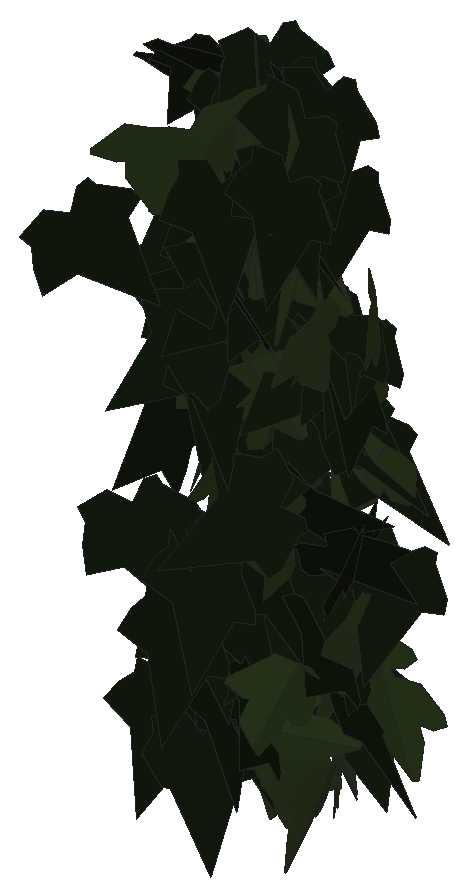
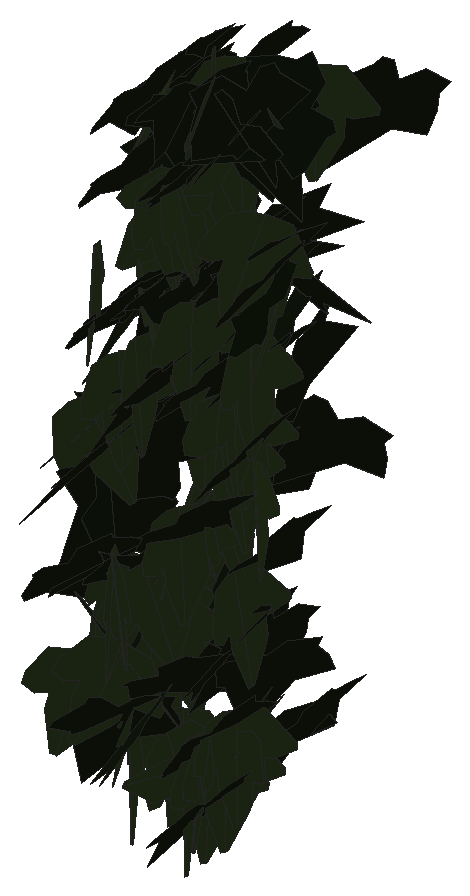
# SketchUp Ruby script. Lengths in inches.
U = 1.inch
M = Sketchup.active_model
def pt(a) = Geom::Point3d.new(a.map { |v| v * U })
def face(e, loops, mat)
  f = e.add_face(loops[0].map { |a| pt(a) })
  loops[1..].each { |l| e.add_face(l.map { |a| pt(a) }).erase! }
  f.material = f.back_material = mat if mat
  f
end
# faces: each face lists its corners as indices into pts; further lists are holes
def faces(e, pts, list, mat = nil) = list.each { |f| face(e, (f[0].is_a?(Array) ? f : [f]).map { |l| l.map { |i| pts[i] } }, mat) }
# xy, xz, yz: faces in a plane at the given z, y or x. An outline is a flat list of corners, or four numbers for a rectangle; further outlines are holes
def ring(l) = l.size == 4 ? [[l[0], l[1]], [l[2], l[1]], [l[2], l[3]], [l[0], l[3]]] : l.each_slice(2).to_a
def flat(e, list, mat, &to3) = list.each { |f| face(e, (f[0].is_a?(Array) ? f : [f]).map { |l| ring(l).map { |u, v| to3.(u, v) } }, mat) }
def xy(e, z, list, mat = nil) = flat(e, list, mat) { |x, y| [x, y, z] }
def xz(e, y, list, mat = nil) = flat(e, list, mat) { |x, z| [x, y, z] }
def yz(e, x, list, mat = nil) = flat(e, list, mat) { |y, z| [x, y, z] }
def lines(e, pts, list) = list.each { |a, b| e.add_line(pt(pts[a]), pt(pts[b])) }
# prism: a flat outline (further loops are holes) pulled along v
def prism(e, loops, v, mat = nil)
  f = face(e, loops, mat); d = Geom::Vector3d.new(v.map { |x| x * U })
  f.pushpull(f.normal.samedirection?(d) ? d.length : -d.length)
end
def box(e, o, s, mat = nil) = prism(e, [[o, [o[0] + s[0], o[1], o[2]], [o[0] + s[0], o[1] + s[1], o[2]], [o[0], o[1] + s[1], o[2]]]], [0, 0, s[2]], mat)
def at(x, y, z, deg = 0) = Geom::Transformation.translation(pt([x, y, z])) * Geom::Transformation.rotation(ORIGIN, Z_AXIS, deg.degrees)
def axes(o, x, y, z) = Geom::Transformation.new([*x, 0, *y, 0, *z, 0, *pt(o).to_a, 1])
def part(name) = M.definitions.add(name)
# library, detail: a bought-in or finely detailed component or shape, given as its bounding box
def library(name, o, s) = part(name).tap { |d| box(d.entities, o, s) }
def detail(e, o, s) = box(e.add_group.entities, o, s)
def put(e, d, t, mat = nil) = e.add_instance(d, t).tap { |i| i.material = mat if mat }
def group(e, t, mat = nil) = e.add_group.tap { |g| g.transformation = t; g.material = mat if mat }.entities
root = M.entities
M.materials.add("efeu1").color = [18, 25, 13]
M.materials.add("efeu2").color = [43, 57, 29]
c1 = part("ivyleaf_10")
p = [[0,0.5,-0.03],[-0.0625,2.02,-0.43],[-0.19,2.01,-0.46],[-0.54,1.05,-0.29],[-0.52,0.625,-0.18],[-0.83,0.76,-0.28],
  [-1.16,0.64,-0.33],[-1.15,0.33,-0.24],[-0.77,-0.39,0.02],[-0.3,-0.51,0.16],[0.04,-0.48,0.23],[-0.02,2.01,-0.4375],
  [-0.06,2.01,-0.43],[0.04,-0.49,0.23],[0.67,-0.49,0.14],[1.38,0.36,-0.2],[1.375,0.51,-0.24],[0.81,0.65,-0.19],
  [0.62,0.59,-0.15],[0.6,1.09,-0.28],[0.5,1.23,-0.31]]
faces(c1.entities,p,[[0,1,2,3,4,5,6,7,8,9,10],[11,12,0,13,14,15,16,17,18,19,20]],"efeu2")
c2 = part("ivyleaf_9")
p = [[1.54,2.16,1.25],[1.36,2.04,1.19],[-0.21,0.99,0.68],[-0.71,1.11,0.82],[-0.85,0.86,0.67],[-0.8,0.17,0.21],
  [-0.9,-0.01,0.1],[-0.67,-0.16,-0.02],[-0.08,-0.08,-0.05],[-0.03,-0.6,-0.4],[0.65,-0.88,-0.66],[0.83,-0.6,-0.49],
  [1.29,-0.42,-0.43],[1.8125,-0.07,-0.26],[1.21,0.44,0.15]]
faces(c2.entities,p,[[0,1,2,3,4,5,6,7,8,9,10,11,12,13,14]],"efeu1")
put(root,c1,axes([19.24,222.77,237.38],[0.17278,-0.38617,-0.2665],[-0.08276,0.25446,-0.42238],[0.46184,0.19007,0.02402]))
put(root,c2,axes([18.98,223.02,240.1],[0.03689,-0.49723,0.03738],[0.00276,-0.03728,-0.4986],[0.49863,0.03699,0]))
put(root,c1,axes([19.14,222.94,240.54],[-0.38375,-0.28732,-0.14208],[0.14647,0.03995,-0.47639],[0.28511,-0.40725,0.0535]))
put(root,c1,axes([19.23,223.1,236.16],[-0.02784,-0.49904,-0.01339],[0.00029,0.01339,-0.49982],[0.49922,-0.02784,-0.00046]))
put(root,c2,axes([18.89,222.41,241.98],[0.46915,0.04238,0.16764],[0.15648,0.10224,-0.46375],[-0.07359,0.4876,0.08267]))
put(root,c2,axes([19.27,222.8,240.12],[-0.27145,-0.32528,0.26553],[-0.08709,-0.2657,-0.41451],[0.41077,-0.27129,0.08759]))
put(root,c2,axes([19.43,222.72,242.08],[0.08196,0.35297,-0.34452],[-0.16723,-0.30867,-0.35603],[-0.46402,0.17359,0.06745]))
put(root,c1,axes([19.3,223.07,234.42],[-0.19485,-0.45862,-0.04129],[0.00891,0.04107,-0.49823],[0.46039,-0.1949,-0.00783]))
put(root,c2,axes([19.64,221.89,239.57],[-0.25149,0.23224,0.36444],[-0.31807,0.18598,-0.338],[-0.29255,-0.40184,0.05419]))
put(root,c2,axes([18.9,223.07,239.83],[0.23492,-0.30149,0.32236],[0.19362,-0.25778,-0.38218],[0.39664,0.30439,-0.00437]))
put(root,c1,axes([19.32,223.25,234.19],[-0.19054,-0.46002,-0.04561],[0.01084,0.04488,-0.49786],[0.46214,-0.19072,-0.00713]))
put(root,c2,axes([19.2,222.13,234.18],[-0.08276,-0.46166,0.17327],[-0.00631,-0.17469,-0.46845],[0.49306,-0.07972,0.02309]))
put(root,c1,axes([19.375,222.71,238.78],[-0.05874,-0.48909,-0.08565],[0.01706,0.0842,-0.49256],[0.49624,-0.06079,0.0068]))
put(root,c1,axes([19.51,222.18,239.29],[-0.08738,0.22127,0.43978],[-0.26336,0.35636,-0.23162],[-0.41594,-0.27212,0.05427]))
put(root,c2,axes([19.2,222.62,235.64],[0.14122,-0.29563,-0.37771],[-0.0462,0.38352,-0.31745],[0.47741,0.12456,0.081]))
put(root,c2,axes([19.24,222.63,235.18],[-0.0934,-0.44065,-0.21703],[0.05724,0.20965,-0.4503],[0.48785,-0.10896,0.01128]))
put(root,c1,axes([19.54,222.79,241.7],[-0.46424,-0.16739,0.08041],[-0.06712,-0.0506,-0.49288],[0.17314,-0.46842,0.02451]))
put(root,c2,axes([19.2,223.3125,235.59],[0.1715,-0.46778,-0.04208],[0.00756,0.04754,-0.49768],[0.46961,0.17007,0.02338]))
put(root,c2,axes([19.27,223.14,237.83],[-0.00405,-0.47425,0.15835],[0.02505,-0.15835,-0.4736],[0.49936,0.0041,0.02504]))
put(root,c2,axes([19.22,223.73,233.86],[0.16797,-0.44931,-0.1411],[0.02929,0.15948,-0.47298],[0.47003,0.15062,0.0799]))
put(root,c1,axes([19.54,221.43,241.57],[-0.40762,-0.28889,0.01977],[-0.01661,-0.01076,-0.49961],[0.28908,-0.40796,-0.00083]))
put(root,c1,axes([19.55,223.18,233.95],[-0.16684,-0.46113,-0.09759],[0.03236,0.09207,-0.49038],[0.47023,-0.16995,-0.00088]))
put(root,c1,axes([19.59,223.3,234.125],[0.28488,-0.29459,-0.28647],[-0.05686,0.31697,-0.38249],[0.40696,0.2505,0.1471]))
put(root,c2,axes([19.4,223.38,234.53],[-0.02239,-0.4995,0.00124],[-0.00344,-0.00109,-0.49999],[0.49949,-0.0224,-0.00339]))
put(root,c2,axes([19.41,220.2,241.14],[0.03149,-0.2267,-0.44454],[0.00486,0.44554,-0.22687],[0.49898,0.00997,0.03026]))
put(root,c1,axes([19.61,222.68,238.23],[0.06106,-0.48381,-0.11043],[0.01791,0.11334,-0.48666],[0.49593,0.05548,0.03117]))
put(root,c1,axes([19.55,222.72,241.24],[0.11348,0.48549,0.03771],[-0.04596,0.04922,-0.49544],[-0.48478,0.10898,0.0558]))
put(root,c2,axes([19.375,222.8125,234.2],[0.24582,-0.43247,-0.05045],[-0.00936,0.05267,-0.49713],[0.4353,0.24535,0.0178]))
put(root,c1,axes([19.77,222.54,237.92],[-0.43303,-0.23228,0.09238],[-0.07562,-0.0544,-0.49125],[0.23827,-0.43941,0.01198]))
put(root,c2,axes([19.41,222.92,241.8],[-0.18122,-0.09721,-0.45575],[0.39386,0.22941,-0.20554],[0.24907,-0.4335,-0.00657]))
put(root,c2,axes([19.47,222.6,235.58],[0.17757,-0.38809,-0.26049],[-0.05617,0.25891,-0.42404],[0.46402,0.17985,0.04835]))
put(root,c2,axes([19.58,222.3,236.23],[-0.10249,-0.4613,0.16341],[-0.02049,-0.16276,-0.47232],[0.48895,-0.10351,0.01446]))
put(root,c1,axes([19.72,223.4,233.85],[0.32472,-0.28577,-0.25078],[-0.07158,0.27795,-0.40941],[0.3734,0.3018,0.1396]))
put(root,c2,axes([19.52,222.65,239.96],[-0.01102,-0.49986,-0.00467],[0.00024,0.00466,-0.49998],[0.49988,-0.01102,0.00014]))
put(root,c2,axes([19.5625,222.9375,241.47],[0.02201,-0.47233,0.16255],[0.00914,-0.1623,-0.47284],[0.49943,0.02379,0.00149]))
put(root,c1,axes([19.82,222.4,237.33],[0.00796,-0.49503,-0.06988],[-0.01366,0.06965,-0.49494],[0.49975,0.00979,-0.01242]))
put(root,c2,axes([19.65,221.61,238.19],[0.0786,-0.17823,-0.46049],[0.3059,-0.34846,0.18709],[-0.38762,-0.31114,0.05426]))
put(root,c2,axes([19.51,221.875,238.9],[0.32,-0.38407,0.00967],[0.00641,-0.00725,-0.49991],[0.38414,0.32006,0.00028]))
put(root,c2,axes([19.63,222.4,238.52],[-0.03097,-0.48134,0.13171],[0.02916,-0.13348,-0.48097],[0.49819,-0.02211,0.03634]))
put(root,c2,axes([19.5625,222.56,234.29],[0.14424,-0.45462,0.15005],[0.02872,-0.14821,-0.47666],[0.47788,0.14613,-0.01664]))
put(root,c2,axes([19.67,222.09,233.92],[-0.07523,-0.47784,-0.12654],[0.0303,0.1233,-0.48361],[0.49338,-0.08043,0.01041]))
put(root,c2,axes([19.6,221,237.25],[-0.11147,-0.25925,-0.41275],[0.2764,0.31513,-0.27258],[0.40147,-0.28893,0.07305]))
put(root,c2,axes([19.83,223.42,236.98],[-0.22323,-0.42942,0.12557],[0.01525,-0.14755,-0.47749],[0.44714,-0.20935,0.07897]))
put(root,c1,axes([19.64,222.12,239.84],[-0.32479,0.06175,-0.3751],[0.34635,-0.15528,-0.32546],[-0.15669,-0.47125,0.0581]))
put(root,c2,axes([19.98,223.5,235.09],[-0.32862,-0.34969,0.14046],[-0.03433,-0.15781,-0.4732],[0.37528,-0.32064,0.07971]))
put(root,c1,axes([19.88,222.84,242.1],[-0.17244,0.40379,-0.23921],[0.07485,-0.22793,-0.43869],[-0.46332,-0.1871,0.01816]))
put(root,c1,axes([20.01,222.4,236.65],[0.0629,-0.48601,0.0992],[0.02876,-0.09625,-0.4898],[0.49519,0.06733,0.01584]))
put(root,c1,axes([19.88,223.01,233.77],[0.12226,0.01737,-0.48451],[0.21946,0.44357,0.07128],[0.43231,-0.23009,0.10084]))
put(root,c1,axes([20.03,222.17,241.58],[-0.04064,-0.42806,-0.25517],[0.0721,0.24827,-0.42798],[0.4931,-0.07158,0.04155]))
put(root,c1,axes([20.09,223.04,236.625],[-0.14708,-0.47659,-0.0351],[0.01122,0.03327,-0.49877],[0.47775,-0.1475,0.0009]))
put(root,c2,axes([19.94,222.94,238.45],[-0.10769,-0.46778,0.13995],[0.01987,-0.14739,-0.47737],[0.48786,-0.09725,0.05033]))
put(root,c2,axes([19.89,223,242.14],[0.04424,-0.45024,-0.21291],[0.02707,0.2156,-0.45031],[0.4973,0.02832,0.04346]))
put(root,c1,axes([20.05,222.08,240.57],[-0.42098,0.25796,-0.07898],[0.07309,-0.03184,-0.4936],[-0.25969,-0.42713,-0.0109]))
put(root,c1,axes([20.08,222.17,241.8],[-0.27717,-0.39435,-0.1329],[0.11239,0.08282,-0.48011],[0.40068,-0.29602,0.04273]))
put(root,c2,axes([20.12,222.04,239.7],[-0.21627,-0.32562,0.31177],[-0.02329,-0.33726,-0.36839],[0.45021,-0.17387,0.13071]))
put(root,c2,axes([20.05,222.95,241.85],[-0.19656,-0.40287,-0.22149],[0.11851,0.18834,-0.44775],[0.44421,-0.22852,0.02145]))
put(root,c1,axes([20.25,222.95,233.77],[-0.07528,-0.48543,0.09321],[-0.0002,-0.09426,-0.49103],[0.4943,-0.07396,0.014]))
put(root,c2,axes([20.3,221.33,239.46],[-0.22843,-0.319,0.30993],[-0.1806,-0.25188,-0.39235],[0.40645,-0.2912,-0.00015]))
put(root,c1,axes([20.31,222.57,238.875],[-0.16578,-0.46461,-0.08156],[0.01192,0.0823,-0.49304],[0.47157,-0.16541,-0.01621]))
put(root,c2,axes([20.01,222.85,241.08],[0.21018,-0.42419,-0.16091],[0.02326,0.18718,-0.46306],[0.45308,0.18716,0.09842]))
put(root,c2,axes([20.16,222.67,239.69],[-0.14333,-0.41614,0.23724],[0.036,-0.25629,-0.42781],[0.47766,-0.10556,0.10343]))
put(root,c1,axes([20.37,222.7,240.54],[0.05537,-0.49655,-0.01922],[-0.01086,0.01813,-0.49955],[0.49681,0.05574,-0.00878]))
put(root,c1,axes([20.43,223.17,235.89],[-0.22569,-0.42262,0.14302],[-0.02015,-0.15045,-0.4764],[0.44571,-0.2208,0.05088]))
put(root,c1,axes([20.49,222.5625,233.8],[-0.46566,-0.17103,0.06249],[-0.05953,-0.01918,-0.49607],[0.17208,-0.46945,-0.0025]))
put(root,c2,axes([20.15,223.65,234.47],[0.26996,-0.41961,-0.03238],[-0.01824,0.02676,-0.49895],[0.42046,0.27058,-0.00086]))
put(root,c2,axes([20.2,222.24,238.47],[0.08146,-0.49264,0.02591],[0.00732,-0.02505,-0.49932],[0.49327,0.08172,0.00313]))
put(root,c1,axes([20.45,222.89,240.53],[-0.08095,-0.49292,0.02187],[0.01292,-0.02427,-0.49924],[0.49324,-0.08026,0.01666]))
put(root,c2,axes([20.21,222.7,240.98],[0.08881,-0.47835,-0.11529],[0.01541,0.1198,-0.48519],[0.49181,0.08263,0.03602]))
put(root,c2,axes([20.28,221.53,239.11],[0.08663,-0.49143,0.03154],[0.00496,-0.03115,-0.499],[0.49241,0.08677,-0.00052]))
put(root,c1,axes([20.48,222.38,236.47],[0.14237,-0.36035,-0.31603],[0.04568,0.33838,-0.36526],[0.47712,0.07513,0.12927]))
put(root,c2,axes([20.31,222.67,239.52],[0.08382,-0.43797,-0.22617],[0.02808,0.23328,-0.44135],[0.49212,0.06129,0.06371]))
put(root,c2,axes([20.4,221.29,236.625],[-0.05643,-0.48836,0.09123],[0.02027,-0.09401,-0.49066],[0.49639,-0.05168,0.0304]))
put(root,c2,axes([20.4375,221.625,239.95],[0.44629,-0.0716,-0.21377],[-0.20932,0.04446,-0.45189],[0.08372,0.49285,0.00971]))
put(root,c1,axes([20.5625,221.86,237.63],[0.21074,-0.44521,0.08587],[0.02404,-0.08359,-0.49238],[0.45278,0.21166,-0.01383]))
put(root,c1,axes([20.57,223.52,236.12],[0.31223,-0.37642,-0.10404],[-0.00976,0.12563,-0.48386],[0.39041,0.30418,0.0711]))
put(root,c2,axes([20.36,222.34,236.25],[0.23697,-0.43101,-0.08987],[-0.02032,0.09124,-0.49118],[0.43981,0.23645,0.02573]))
put(root,c2,axes([20.39,223.03,238.43],[0.24888,-0.34968,-0.25648],[-0.06132,0.26436,-0.41994],[0.4293,0.24049,0.0887]))
put(root,c1,axes([20.64,223.48,235.95],[0.1365,-0.42725,-0.22097],[0.00098,0.22994,-0.44399],[0.48101,0.12077,0.06361]))
put(root,c2,axes([20.51,220.74,236.26],[-0.06199,-0.4858,0.10077],[-0.0083,-0.10052,-0.48972],[0.49607,-0.06239,0.0044]))
put(root,c1,axes([20.65,222.2,238.55],[0.01428,-0.47018,0.16949],[0.05129,-0.16729,-0.46838],[0.49716,0.03077,0.04345]))
put(root,c1,axes([20.6875,222.37,234.85],[-0.01684,-0.49028,0.09666],[0.00078,-0.09675,-0.49055],[0.49972,-0.01637,0.00402]))
put(root,c1,axes([20.62,221.89,238.875],[-0.38719,-0.2451,-0.20004],[0.16377,0.11522,-0.45815],[0.27068,-0.4203,-0.00894]))
put(root,c1,axes([20.73,222.96,238.45],[0.08262,-0.48164,-0.10582],[0.00343,0.10786,-0.48822],[0.49311,0.07995,0.02113]))
put(root,c1,axes([20.73,223.06,233.74],[0.30665,-0.3399,-0.20109],[-0.03357,0.23123,-0.44205],[0.3935,0.28461,0.11899]))
put(root,c1,axes([20.79,221.7,237.35],[-0.20833,-0.44843,-0.07421],[0.0183,0.07329,-0.49426],[0.45416,-0.20865,-0.01412]))
put(root,c2,axes([20.61,223.09,236.16],[-0.13064,-0.47787,-0.06764],[0.09056,0.04456,-0.48971],[0.47406,-0.1402,0.07491]))
put(root,c2,axes([20.64,221.21,241.47],[0.00137,-0.49923,-0.02763],[-0.00107,0.02763,-0.49924],[0.5,0.00142,-0.001]))
put(root,c1,axes([20.79,222.92,234.22],[-0.25424,0.42516,0.0678],[-0.01962,0.06721,-0.49507],[-0.43009,-0.2544,-0.01749]))
put(root,c2,axes([20.64,223.44,234.41],[-0.09193,-0.40844,-0.27336],[0.11421,0.25274,-0.41603],[0.47802,-0.13893,0.04682]))
put(root,c2,axes([20.78,222.8,238.12],[-0.21671,-0.43546,0.11579],[-0.00565,-0.12585,-0.48387],[0.45056,-0.21103,0.04963]))
put(root,c1,axes([20.77,223.34,234.87],[-0.4298,-0.17652,-0.18469],[0.17822,0.05181,-0.46428],[0.18304,-0.46493,0.01838]))
put(root,c1,axes([20.71,222.31,240.2],[-0.32433,-0.2441,-0.29193],[0.25927,0.13902,-0.40429],[0.27854,-0.41363,0.0364]))
put(root,c2,axes([20.69,222.96,241.86],[0.02096,-0.49886,-0.02644],[-0.0003,0.02645,-0.4993],[0.49956,0.02095,0.00081]))
put(root,c1,axes([20.92,222.58,239.24],[0.17646,-0.45863,-0.09228],[-0.03724,0.08454,-0.49139],[0.46634,0.1803,-0.00433]))
put(root,c1,axes([20.82,222.28,240.22],[0.346,-0.35122,0.08326],[0.05491,-0.06277,-0.493],[0.35675,0.35029,-0.00487]))
put(root,c1,axes([20.95,223,238.22],[-0.1625,-0.47023,-0.04974],[0.01155,0.04864,-0.49749],[0.47271,-0.16284,-0.00494]))
put(root,c1,axes([20.83,222.27,241.63],[0.21491,-0.32125,-0.3172],[0.1054,0.3773,-0.3107],[0.43898,0.06668,0.22989]))
put(root,c2,axes([20.79,222.43,241.81],[-0.1005,-0.46062,0.16653],[0.01475,-0.17277,-0.46897],[0.48957,-0.08936,0.04831]))
put(root,c2,axes([21.26,222.91,234.99],[-0.3338,0.31581,0.19708],[-0.15085,0.12724,-0.45941],[-0.34032,-0.36616,0.01034]))
put(root,c2,axes([20.98,222.6,238.97],[-0.30259,-0.33094,0.22118],[-0.05735,-0.23869,-0.43559],[0.39389,-0.28898,0.10649]))
put(root,c2,axes([20.58,222.2,240.88],[0.31279,-0.33988,0.19142],[0.16108,-0.11092,-0.46016],[0.35527,0.34953,0.0401]))
put(root,c2,axes([20.79,221.7,234.83],[0.00847,-0.26597,0.42331],[0.0393,-0.4217,-0.26575],[0.49838,0.03777,0.01376]))
put(root,c2,axes([20.875,223.06,240.88],[-0.05455,-0.48617,0.10325],[-0.00344,-0.1035,-0.48916],[0.497,-0.05407,0.00795]))
put(root,c2,axes([20.95,223.04,239.16],[-0.14454,-0.43844,0.19205],[-0.01513,-0.19633,-0.45959],[0.47841,-0.13867,0.04349]))
put(root,c2,axes([20.875,221.98,241.48],[0.07605,-0.47848,-0.12359],[0.0104,0.12657,-0.4836],[0.49407,0.07099,0.0292]))
put(root,c1,axes([21.13,222.78,235.09],[-0.02255,-0.49778,0.04137],[-0.0067,-0.0411,-0.49826],[0.49945,-0.02303,-0.00482]))
put(root,c1,axes([21.33,223.04,237.58],[-0.39509,-0.15053,0.26691],[-0.22777,-0.14709,-0.4201],[0.205,-0.45355,0.04766]))
put(root,c2,axes([20.6875,222.42,237.05],[0.17416,-0.17044,0.4366],[0.40834,-0.17345,-0.2306],[0.23006,0.43688,0.07878]))
put(root,c2,axes([21.02,223.15,239.05],[-0.10707,-0.45785,0.17004],[0.01325,-0.17674,-0.46753],[0.48822,-0.09561,0.04998]))
put(root,c2,axes([20.89,223.03,238.03],[0.30156,-0.35263,-0.18632],[-0.01972,0.22012,-0.44851],[0.39834,0.27785,0.11885]))
put(root,c2,axes([20.91,223.36,237.52],[0.27372,-0.35333,-0.22414],[-0.02259,0.25497,-0.42951],[0.41782,0.24525,0.12362]))
put(root,c1,axes([20.95,221.71,234.71],[-0.14301,-0.14728,-0.45591],[0.35692,0.28466,-0.20391],[0.31962,-0.38377,0.02372]))
put(root,c2,axes([21.01,222.63,235.36],[-0.06975,-0.29293,0.39916],[0.08596,-0.40415,-0.28156],[0.48759,0.02934,0.10674]))
put(root,c2,axes([21.06,222.59,236.5625],[0.43347,0.24526,0.04422],[0.03866,0.02147,-0.49804],[-0.24619,0.43519,-0.00035]))
put(root,c1,axes([21.21,222.7,235.5625],[-0.03843,-0.42115,-0.26676],[0.08195,0.25857,-0.42003],[0.49174,-0.076,0.04915]))
put(root,c2,axes([21.52,221.03,237.92],[-0.46433,-0.08126,0.1667],[-0.16177,-0.04227,-0.47121],[0.09068,-0.49154,0.01297]))
put(root,c2,axes([21.11,221.78,241.41],[-0.03757,-0.48527,0.11447],[-0.0177,-0.11343,-0.48664],[0.49827,-0.04062,-0.00866]))
put(root,c1,axes([21.3125,221.48,235.48],[-0.16721,-0.37488,0.28549],[0.01298,-0.30649,-0.39484],[0.47103,-0.12463,0.11223]))
put(root,c1,axes([21.25,222.14,233.92],[0.10909,-0.4271,0.23598],[0.06874,-0.22594,-0.44071],[0.48309,0.1286,0.00942]))
put(root,c2,axes([21.14,222.71,236.08],[0.06384,0.38842,0.30831],[-0.06615,-0.3014,0.39342],[0.49148,-0.09102,0.0129]))
put(root,c1,axes([21.25,223.04,239.43],[0.28325,-0.38921,-0.13523],[0.0466,0.19331,-0.45876],[0.40939,0.24728,0.14579]))
put(root,c2,axes([21.21,223.55,236.06],[-0.1678,-0.46983,0.03319],[0.00139,-0.03573,-0.49872],[0.471,-0.16728,0.0133]))
put(root,c2,axes([21.08,222.91,238.61],[0.0736,-0.42294,0.25632],[0.04539,-0.25227,-0.4293],[0.49247,0.08647,0.00126]))
put(root,c1,axes([21.36,221.84,239.68],[0.00098,-0.4654,-0.18276],[0.05143,0.18188,-0.4629],[0.49735,-0.01789,0.04823]))
put(root,c2,axes([21.06,222.9,234.5625],[0.33818,-0.36674,0.03371],[0.03119,-0.01708,-0.49873],[0.36696,0.33943,0.01133]))
put(root,c1,axes([21.33,223.3,234.52],[-0.49047,-0.03469,-0.09077],[0.09463,-0.06422,-0.48675],[0.02212,-0.49464,0.06956]))
